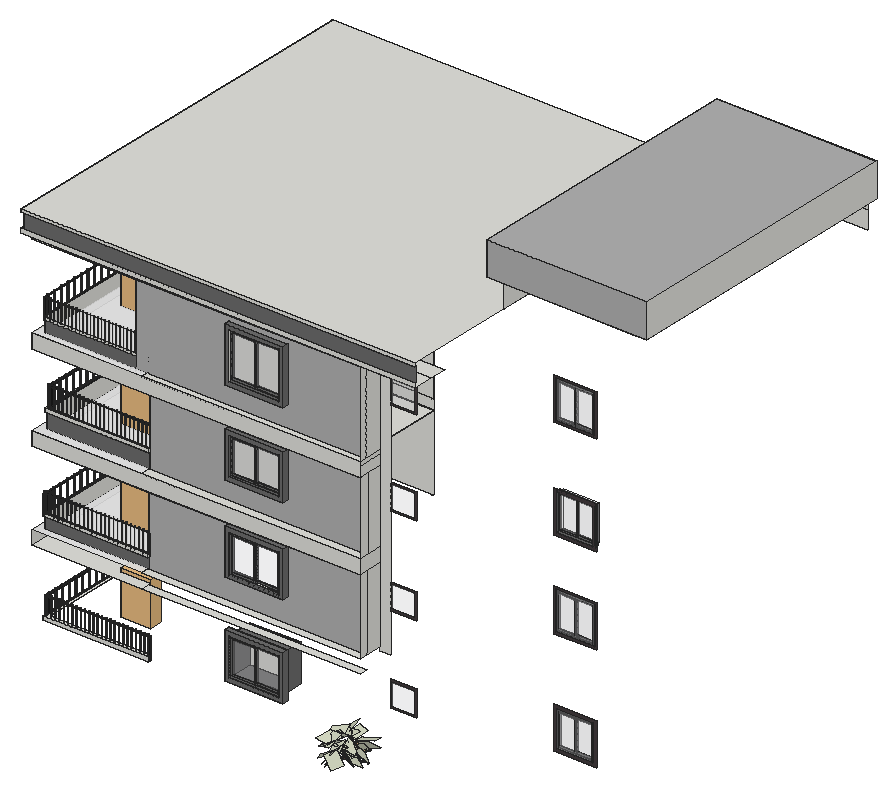
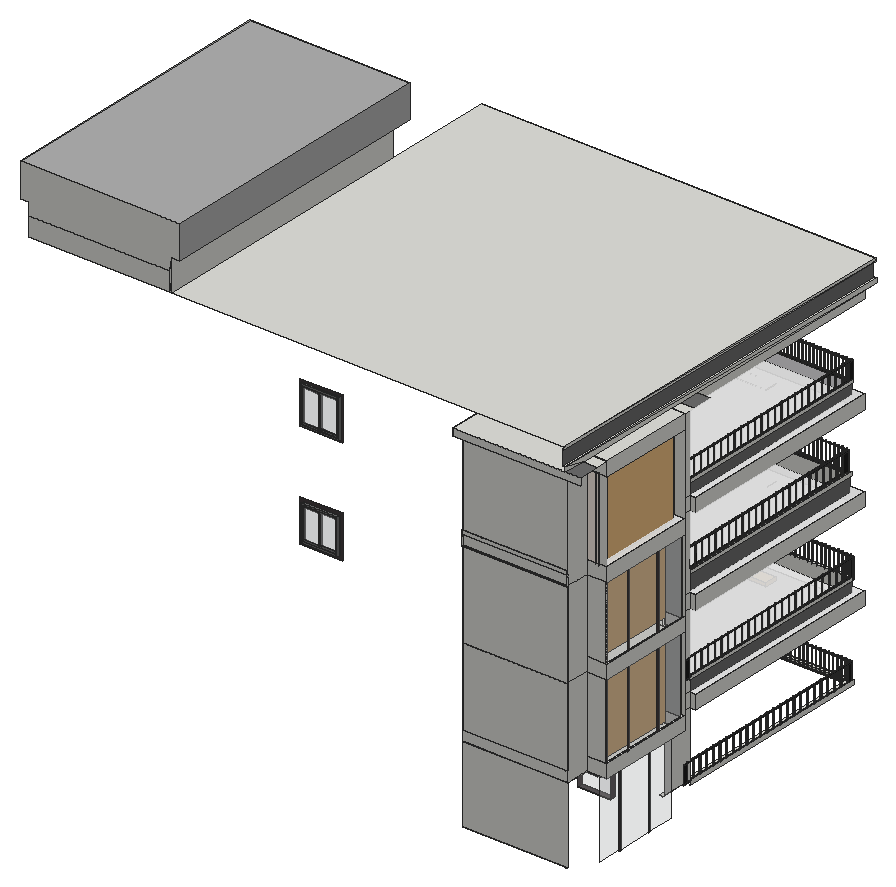
# SketchUp Ruby script. Lengths in inches.
U = 1.inch
M = Sketchup.active_model
def pt(a) = Geom::Point3d.new(a.map { |v| v * U })
def face(e, loops, mat)
  f = e.add_face(loops[0].map { |a| pt(a) })
  loops[1..].each { |l| e.add_face(l.map { |a| pt(a) }).erase! }
  f.material = f.back_material = mat if mat
  f
end
# faces: each face lists its corners as indices into pts; further lists are holes
def faces(e, pts, list, mat = nil) = list.each { |f| face(e, (f[0].is_a?(Array) ? f : [f]).map { |l| l.map { |i| pts[i] } }, mat) }
# xy, xz, yz: faces in a plane at the given z, y or x. An outline is a flat list of corners, or four numbers for a rectangle; further outlines are holes
def ring(l) = l.size == 4 ? [[l[0], l[1]], [l[2], l[1]], [l[2], l[3]], [l[0], l[3]]] : l.each_slice(2).to_a
def flat(e, list, mat, &to3) = list.each { |f| face(e, (f[0].is_a?(Array) ? f : [f]).map { |l| ring(l).map { |u, v| to3.(u, v) } }, mat) }
def xy(e, z, list, mat = nil) = flat(e, list, mat) { |x, y| [x, y, z] }
def xz(e, y, list, mat = nil) = flat(e, list, mat) { |x, z| [x, y, z] }
def yz(e, x, list, mat = nil) = flat(e, list, mat) { |y, z| [x, y, z] }
def lines(e, pts, list) = list.each { |a, b| e.add_line(pt(pts[a]), pt(pts[b])) }
# prism: a flat outline (further loops are holes) pulled along v
def prism(e, loops, v, mat = nil)
  f = face(e, loops, mat); d = Geom::Vector3d.new(v.map { |x| x * U })
  f.pushpull(f.normal.samedirection?(d) ? d.length : -d.length)
end
def box(e, o, s, mat = nil) = prism(e, [[o, [o[0] + s[0], o[1], o[2]], [o[0] + s[0], o[1] + s[1], o[2]], [o[0], o[1] + s[1], o[2]]]], [0, 0, s[2]], mat)
def at(x, y, z, deg = 0) = Geom::Transformation.translation(pt([x, y, z])) * Geom::Transformation.rotation(ORIGIN, Z_AXIS, deg.degrees)
def axes(o, x, y, z) = Geom::Transformation.new([*x, 0, *y, 0, *z, 0, *pt(o).to_a, 1])
def part(name) = M.definitions.add(name)
# library, detail: a bought-in or finely detailed component or shape, given as its bounding box
def library(name, o, s) = part(name).tap { |d| box(d.entities, o, s) }
def detail(e, o, s) = box(e.add_group.entities, o, s)
def put(e, d, t, mat = nil) = e.add_instance(d, t).tap { |i| i.material = mat if mat }
def group(e, t, mat = nil) = e.add_group.tap { |g| g.transformation = t; g.material = mat if mat }.entities
root = M.entities
M.materials.add("Celtis_australis_s cópia1").color = [224, 229, 205]
M.materials.add("Niraj_Hair_Dark").color = [109, 109, 109]
M.materials.add("Niraj_Hair_Gray").color = [178, 178, 178]
M.materials.add("Tendaggio").color = [239, 239, 239]
M.materials["Tendaggio"].alpha = 0.9
M.materials.add("[0009_Linen]").color = [250, 240, 230]
M.materials.add("[Asphalt New]").color = [67, 60, 62]
M.materials.add("[Color M08]").color = [30, 30, 30]
M.materials.add("[CoolGray4]").color = [225, 226, 230]
M.materials["[CoolGray4]"].alpha = 0.26
M.materials.add("aubin blanc").color = [238, 236, 240]
M.materials.add("bark_cherry").color = [99, 76, 62]
c1 = part("branch2\#1")
p = [[13.74,0.36,0.5],[11.5,11.3125,10.98],[14.125,0.95,0],[14.97,0.95,0.19],[12.12,10.6875,11.67],[15.1,0.36,0.82],
  [11.05,10.4375,11.49],[14.34,0,1.01],[6.08,18.54,23.51],[6.83,18.32,23.89],[6.09,17.93,24.13],[3.27,29.37,34],
  [3.27,29.68,33.56],[3.73,29.59,33.82],[0,43.16,40.74],[0,43.16,40.75],[0.01,43.16,40.75],[5.59,23.2,32.77],
  [4.65,30.48,39.08],[1.92,39.79,43.02],[5.09,28.47,41.41]]
faces(c1.entities,p,[[0,1,2],[2,1,3],[3,4,5],[3,1,4],[6,0,7],[0,6,1],[5,6,7],[6,5,4],
  [6,8,1],[1,9,4],[9,1,8],[8,6,10],[4,10,6],[10,4,9],[10,11,8],[8,12,9],
  [12,8,11],[10,9,11],[13,11,9],[13,9,12],[14,12,11,15],[12,14,16,13],[13,16,15,11]],"bark_cherry")
lines(c1.entities,p,[[17,18],[11,19],[20,17],[17,10]])
c2 = part("branch3")
p = [[6.085,7.082,2.644],[4.083,0.001,0],[4.08,0.002,0.001],[5.841,7.141,2.739],[4.083,0,0.004],[6.032,7.035,2.901],
  [8.234,14.378,3.666],[10.055,21.673,1.937],[8.611,14.241,3.496],[10.247,21.661,2.456],[9.737,21.9,2.346],[9.715,21.803,2.365],
  [12.357,28.999,2.225],[12.894,28.763,2.608],[12.761,28.844,2.204],[10.064,22.087,2.083],[10.362,21.9,2.346],[5.434,16.028,3.111],
  [10.04,22.14,2.516],[12.239,29.014,2.642],[8.553,14.232,3.928],[5.628,15.927,3.273],[5.444,16.098,3.367],[12.571,28.869,2.879],
  [0.628,10.534,6.01],[0.625,10.536,6.008],[0.625,10.537,6.012],[6.135,9.846,4.735],[0.003,10.534,6.01],[0,10.537,6.012],
  [1.761,10.232,4.093],[4.16,5.476,4.049],[3.718,5.459,5.543],[3.205,0.783,1.919]]
faces(c2.entities,p,[[0,1,2,3],[3,2,4,5],[1,0,5,4],[6,7,8],[9,8,7],[7,6,10,11],[12,7,11],[13,7,14],
  [14,7,12],[13,9,7],[15,16,17],[15,17,18],[12,11,19],[20,10,6],[10,20,9,11],[21,17,16],
  [21,16,22],[18,22,16],[9,19,11],[8,9,20],[22,18,17],[9,13,23],[19,9,23],[0,8,5],
  [3,6,0],[8,0,6],[3,5,6],[20,5,8],[20,6,5],[21,24,25,17],[26,22,17,25],[22,26,24,21]],"bark_cherry")
lines(c2.entities,p,[[27,20],[28,29],[17,30],[27,31],[32,27],[5,33]])
c3 = part("leaf1\#1")
p = [[1.6,6.78,0.04],[-9.34,-4.04,0.02],[2.67,-16.2,2.05],[13.62,-5.38,2.07]]
faces(c3.entities,p,[[0,1,2,3]],"Celtis_australis_s cópia1")
c4 = part("leaf_group1\#1")
put(c4.entities,c3,axes([-0.06,3.68,7.3125],[0.53029,-0.80282,-0.27253],[0.82812,0.42159,0.36943],[-0.18168,-0.42159,0.8884]))
put(c4.entities,c3,axes([6.4375,-3.58,5.23],[1,0,0],[0,0.98927,0.14608],[0,-0.14608,0.98927]))
put(c4.entities,c3,axes([-0.99,3.68,1.22],[0.57591,-0.80282,0.15431],[0.36532,0.42159,0.82994],[-0.73135,-0.42159,0.53609]))
put(c4.entities,c3,axes([18.71,8.59,4.39],[0.33053,0.77491,0.53877],[-0.79988,-0.073,0.5957],[0.50094,-0.62785,0.5957]))
put(c4.entities,c3,axes([13.16,0.76,0.89],[0.89618,0.3501,0.27256],[-0.44248,0.65988,0.60727],[0.03275,-0.66482,0.74628]))
put(c4.entities,c3,axes([4.53,7.98,7.3125],[-0.1927,0.94265,-0.27253],[0.88368,0.28746,0.36943],[-0.42658,0.16964,0.8884]))
put(c4.entities,c3,axes([12.46,21.28,7.16],[0.85019,0.38493,0.35918],[0.30538,-0.91629,0.25914],[-0.42887,0.11063,0.89657]))
put(c4.entities,c3,axes([6.53,15.18,2.59],[0.70711,0.70711,0],[0.5,-0.5,0.70711],[-0.5,0.5,0.70711]))
put(c4.entities,c3,axes([-3.17,8.15,3.46],[-0.03719,0.74973,0.66069],[0.94096,-0.19634,0.27576],[-0.33647,-0.63194,0.69817]))
put(c4.entities,c3,axes([23.03,17.79,4.39],[0.78166,-0.31422,0.53877],[-0.61722,-0.51398,0.5957],[-0.08973,0.79818,0.5957]))
put(c4.entities,c3,axes([14.78,21.52,3.21],[0.67246,-0.04394,0.73882],[-0.28657,-0.93583,0.20517],[-0.6824,0.3497,0.64191]))
put(c4.entities,c3,axes([10.37,-1.8125,9],[0.99279,-0.06448,-0.101],[0.11527,0.74421,0.65792],[0.03275,-0.66482,0.74628]))
put(c4.entities,c3,axes([1.45,16.1875,2.9375],[-0.2106,-0.86579,-0.45394],[0.96054,-0.26957,0.06852],[-0.18168,-0.42159,0.8884]))
c5 = part("branch1\#1")
p = [[23.875,19.65,51.47],[23.47,20.4,51.62],[21.1,21.64,19.5],[21.93,21.1875,19.92],[21.95,22.18,19.69],[26.48,9.62,42.86],
  [30.79,16.22,49.68],[31.01,4.77,55.38],[31.01,0,68.57],[9.91,24.21,59.69],[9.92,24.21,59.7],[24,20.54,51.64],
  [12.85,4.92,53.79],[26.1,8.92,42.74],[31.84,25.13,88.91],[31.84,25.13,106.45],[30.18,33.29,93.95],[30.18,25.42,69.53],
  [0,6.37,81.52],[11.1,10.75,77.87]]
lines(c5.entities,p,[[0,1],[2,3],[3,4],[5,6],[7,8],[9,10],[1,11],[11,0],[12,13],[4,2],[14,15],[16,17],
  [18,19]])
detail(c5.entities,[5.26,2.24,0],[28.14,24.14,108.01])
c6 = part("Group\#428")
prism(c6.entities,[[[0,1.97,0],[0,1.97,1.18],[0,0,1.18],[0,0,0]],[[0,1.92,1.13],[0,1.92,0.05],[0,0.05,0.05],[0,0.05,1.13]]],[98.43,0,0])
c7 = part("Group\#430")
xy(c7.entities,0,[[0.3,0,0.22,0.01,0.15,0.04,0.09,0.09,0.04,0.15,0.01,0.22,0,0.3,0.3,0.3],[0.3,0,0.3,0.3,0.59,0.3,0.58,0.22,0.55,0.15,0.5,0.09,0.44,0.04,0.37,0.01],[0,0.3,0.01,0.37,0.04,0.44,0.09,0.5,0.15,0.55,0.22,0.58,0.3,0.59,0.3,0.3],[0.3,0.3,0.3,0.59,0.37,0.58,0.44,0.55,0.5,0.5,0.55,0.44,0.58,0.37,0.59,0.3]])
xy(c7.entities,39.37,[[0.3,0,0.37,0.01,0.44,0.04,0.5,0.09,0.55,0.15,0.58,0.22,0.59,0.3,0.58,0.37,0.55,0.44,0.5,0.5,0.44,0.55,0.37,0.58,0.3,0.59,0.22,0.58,0.15,0.55,0.09,0.5,0.04,0.44,0.01,0.37,0,0.3,0.01,0.22,0.04,0.15,0.09,0.09,0.15,0.04,0.22,0.01]])
p = [[0.09,0.09,0],[0.15,0.04,0],[0.15,0.04,39.37],[0.09,0.09,39.37],[0.22,0.01,0],[0.22,0.01,39.37],
  [0.3,0,0],[0.3,0,39.37],[0.37,0.01,0],[0.37,0.01,39.37],[0.44,0.04,0],[0.44,0.04,39.37],
  [0.5,0.09,0],[0.5,0.09,39.37],[0.01,0.22,0],[0.04,0.15,0],[0.04,0.15,39.37],[0.01,0.22,39.37],
  [0.55,0.15,0],[0.55,0.15,39.37],[0.58,0.22,0],[0.58,0.22,39.37],[0,0.3,0],[0,0.3,39.37],
  [0.59,0.3,0],[0.59,0.3,39.37],[0.01,0.37,0],[0.01,0.37,39.37],[0.58,0.37,0],[0.58,0.37,39.37],
  [0.09,0.5,0],[0.04,0.44,0],[0.04,0.44,39.37],[0.09,0.5,39.37],[0.55,0.44,0],[0.5,0.5,0],
  [0.5,0.5,39.37],[0.55,0.44,39.37],[0.15,0.55,0],[0.15,0.55,39.37],[0.44,0.55,0],[0.44,0.55,39.37],
  [0.22,0.58,0],[0.22,0.58,39.37],[0.3,0.59,0],[0.3,0.59,39.37],[0.37,0.58,0],[0.37,0.58,39.37]]
faces(c7.entities,p,[[0,1,2,3],[1,4,5,2],[4,6,7,5],[6,8,9,7],[8,10,11,9],[10,12,13,11],[14,15,16,17],[15,0,3,16],
  [12,18,19,13],[18,20,21,19],[22,14,17,23],[20,24,25,21],[26,22,23,27],[24,28,29,25],[30,31,32,33],[31,26,27,32],
  [34,35,36,37],[28,34,37,29],[38,30,33,39],[35,40,41,36],[42,38,39,43],[44,42,43,45],[46,44,45,47],[40,46,47,41]])
c8 = part("Group\#429")
prism(c8.entities,[[[0.01,0.22,35.83],[0,0.3,35.83],[0.01,0.37,35.83],[0.04,0.44,35.83],[0.09,0.5,35.83],[0.15,0.55,35.83],[0.22,0.58,35.83],[0.3,0.59,35.83],[0.37,0.58,35.83],[0.44,0.55,35.83],[0.5,0.5,35.83],[0.55,0.44,35.83],[0.58,0.37,35.83],[0.59,0.3,35.83],[0.58,0.22,35.83],[0.55,0.15,35.83],[0.5,0.09,35.83],[0.44,0.04,35.83],[0.37,0.01,35.83],[0.3,0,35.83],[0.22,0.01,35.83],[0.15,0.04,35.83],[0.09,0.09,35.83],[0.04,0.15,35.83]]],[0,0,3.54])
c9 = part("Balcony railing panel")
g1 = group(c9.entities,at(0,0,0))
put(g1,c6,axes([0,0,39.76],[1,0,0],[0,0,-1],[0,1,0]),"[Color M08]")
put(g1,c6,axes([0,0,1.97],[1,0,0],[0,0,-1],[0,1,0]),"[Color M08]")
put(g1,c6,axes([98.43,0,37.8],[0,0,-0.364],[-1,0,0],[0,1,0]),"[Color M08]")
put(g1,c6,axes([1.97,0,37.8],[0,0,-0.364],[-1,0,0],[0,1,0]),"[Color M08]")
g2 = group(c9.entities,at(1.67,0.3,1.97))
put(g2,c7,at(78.74,0,0),"[Color M08]")
put(g2,c7,at(90.55,0,0),"[Color M08]")
put(g2,c7,at(82.68,0,0),"[Color M08]")
put(g2,c7,at(86.61,0,0),"[Color M08]")
put(g2,c7,at(66.93,0,0),"[Color M08]")
put(g2,c7,at(11.8125,0,0),"[Color M08]")
put(g2,c7,at(15.75,0,0),"[Color M08]")
put(g2,c7,at(47.24,0,0),"[Color M08]")
put(g2,c7,at(59.06,0,0),"[Color M08]")
put(g2,c8,at(0,0,0),"[Color M08]")
put(g2,c7,at(39.37,0,0),"[Color M08]")
put(g2,c7,at(62.99,0,0),"[Color M08]")
put(g2,c7,at(55.12,0,0),"[Color M08]")
put(g2,c7,at(19.69,0,0),"[Color M08]")
put(g2,c7,at(35.43,0,0),"[Color M08]")
put(g2,c7,at(7.875,0,0),"[Color M08]")
put(g2,c7,at(23.62,0,0),"[Color M08]")
put(g2,c7,at(31.5,0,0),"[Color M08]")
put(g2,c7,at(43.31,0,0),"[Color M08]")
put(g2,c7,at(27.56,0,0),"[Color M08]")
put(g2,c7,at(3.9375,0,0),"[Color M08]")
put(g2,c7,at(51.18,0,0),"[Color M08]")
put(g2,c7,at(70.87,0,0),"[Color M08]")
put(g2,c7,at(74.8,0,0),"[Color M08]")
put(g2,c8,at(94.49,0,0),"[Color M08]")
c10 = part("Window sash")
g3 = group(c10.entities,at(0.98,0,0),"Niraj_Hair_Dark")
prism(g3,[[[-0.98,0,0],[30.98,0,0],[30.98,0,45.6],[-0.98,0,45.6]],[[29.01,0,43.625],[29.01,0,1.97],[0.98,0,1.97],[0.98,0,43.625]]],[0,1.18,0])
g4 = group(c10.entities,at(1.97,0.59,1.97))
xz(g4,0,[[0,0,28.03,41.66]],"[CoolGray4]")
c11 = part("Twin sash window")
put(c11.entities,c10,at(31.97,2.82,1.97))
put(c11.entities,c10,at(1.97,1.25,1.97))
g5 = group(c11.entities,at(0,0,0),"Niraj_Hair_Dark")
prism(g5,[[[65.9,4.72,0],[0,4.72,0],[0,4.72,49.53],[65.9,4.72,49.53]],[[1.97,4.72,47.5625],[1.97,4.72,1.97],[63.93,4.72,1.97],[63.93,4.72,47.5625]]],[0,-4.72,0])
c12 = library("Plane01\#1",[-62.23,-4.43,-95.54],[61.02,8.86,95.65])
c13 = library("Tenda",[0,0,0],[9.09,66.93,111.26])
c14 = library("fronceur+aubin+blanc+(3)",[-47.99,-0.29,1.66],[95.37,4.84,114.09])
xy(root,221.21,[[544.51,339.47,577.96,344.47]],"[Asphalt New]")
xy(root,224.0625,[[500.29,454.11,605.23,454.18]])
xy(root,231.41,[[499.48,97,499.48,301.21,500.29,301.21,500.29,97.6875,605.23,97.6875,605.23,97]])
xy(root,235.75,[[499.48,97,605.23,97,605.23,100.3125,503.33,100.3125,503.33,335.4,500.29,335.4,500.29,301.21,499.48,301.21]])
xy(root,245.54,[[686.26,91.1875,745.01,96.375]],"Niraj_Hair_Dark")
xy(root,249.54,[[690.26,91.1875,741.01,118.125]],"Niraj_Hair_Dark")
xy(root,285,[[544.51,339.47,577.96,344.47]],"[Asphalt New]")
xy(root,287.23,[[690.26,91.1875,741.01,118.125]],"Niraj_Hair_Dark")
xy(root,287.65,[[541.86,336.16,580.61,339.47]])
xy(root,291.23,[[686.26,91.1875,745.01,96.375]],"Niraj_Hair_Dark")
xy(root,299.625,[[488.54,336.16,605.23,336.16,605.23,454.11,500.29,454.11,500.29,430.89,488.54,430.89]])
xy(root,300.47,[[494.79,89.375,494.79,301.21,500.29,301.21,500.29,333.01,479.54,333.01,479.54,430.89,500.29,430.89,500.29,454.11,605.23,454.11,605.23,89.375],[605.23,89.375,823.9,97.6875]])
xy(root,310.625,[[500.29,454.11,605.23,454.49]])
xy(root,314.1875,[[605.23,89.375,823.9,97.3125]])
xy(root,314.1875,[[494.79,89.375,605.23,89.375,605.23,97.3125,500.73,97.3125,500.73,301.21,502.61,301.21,502.61,98.8125,605.23,98.8125,605.23,336.16,580.61,336.16,580.61,341.72,541.86,341.72,541.86,336.16,481.17,336.16,481.17,430.89,479.54,430.89,479.54,333.01,500.29,333.01,500.29,301.21,494.79,301.21]],"Tendaggio")
xy(root,325.23,[[499.98,96.5,605.23,97.3125],[499.98,97.3125,500.73,301.21]])
xy(root,328.3125,[[499.98,96.5,605.23,96.5,605.23,98.8125,502.61,98.8125,502.61,301.21,499.98,301.21]])
xy(root,338.8,[[686.26,91.1875,745.01,96.375]],"Niraj_Hair_Dark")
xy(root,342.8,[[690.26,91.1875,741.01,97.3125]])
xy(root,380.29,[[690.26,91.1875,741.01,97.3125]])
xy(root,381.08,[[541.86,336.16,580.61,341.72]])
xy(root,384.29,[[686.26,91.1875,745.01,96.375]],"Niraj_Hair_Dark")
xy(root,389.4,[[494.79,89.375,494.79,301.21,500.29,301.21,500.29,333.01,479.54,333.01,479.54,430.89,481.17,430.89,481.17,336.16,605.23,336.16,605.23,89.375],[605.23,89.375,823.9,97.3125],[605.23,97.3125,823.9,113.9375],[481.17,336.16,605.23,336.16,605.23,454.11,500.29,454.11,500.29,430.89,481.17,430.89],[500.29,454.11,605.23,454.49]])
xy(root,403.5,[[605.23,89.375,823.9,98.6875],[605.23,98.6875,823.9,113.9375]])
xy(root,403.5,[[494.79,89.375,605.23,89.375,605.23,98.6875,501.67,98.6875,501.67,301.21,502.78,301.21,502.78,99.8125,605.23,99.8125,605.23,336.16,580.61,336.16,580.61,338.78,541.86,338.78,541.86,336.16,480.73,336.16,480.73,430.89,479.54,430.89,479.54,333.01,500.29,333.01,500.29,301.21,494.79,301.21]],"Tendaggio")
xy(root,404.95,[[543.31,338.78,579.16,338.78,579.16,339.47],[543.31,338.78,579.16,339.47,543.31,339.47]],"[Asphalt New]")
xy(root,419.01,[[501.11,97.6875,501.67,301.21],[501.67,97.6875,605.23,98.6875]])
xy(root,422.125,[[501.11,97.6875,605.23,97.6875,605.23,99.8125,502.78,99.8125,502.78,301.21,501.11,301.21]])
xy(root,425.67,[[686.26,91.1875,745.01,96.375]],"Niraj_Hair_Dark")
xy(root,426.12,[[942.54,187.625,978.5,195.5]],"[CoolGray4]")
xy(root,429.67,[[690.26,91.1875,741.01,96.375]])
xy(root,462.08,[[942.54,187.625,978.5,195.5]],"[CoolGray4]")
xy(root,466.04,[[543.31,338.78,543.31,339.47,579.16,339.47],[543.31,338.78,579.16,339.47,579.16,338.78]],"[Asphalt New]")
xy(root,467.36,[[690.26,91.1875,741.01,96.375]],"Niraj_Hair_Dark")
xy(root,467.49,[[541.86,336.16,580.61,338.78]],"[Asphalt New]")
xy(root,471.36,[[686.26,91.1875,745.01,96.375]],"Niraj_Hair_Dark")
xy(root,476.89,[[494.79,89.375,494.79,301.21,500.29,301.21,500.29,333.01,479.54,333.01,479.54,430.89,480.73,430.89,480.73,336.16,605.23,336.16,605.23,89.375],[605.23,89.375,823.9,98.6875],[605.23,98.6875,823.9,113.9375],[480.73,336.16,605.23,336.16,605.23,454.49,500.29,454.49,500.29,430.89,480.73,430.89],[500.29,454.49,605.23,455.3]])
xy(root,490.8125,[[605.23,89.375,823.9,96.375],[605.23,96.375,823.9,96.375,823.9,113.9375,593.42,113.9375,593.42,96.75,605.23,96.75],[593.42,113.9375,605.23,336.16],[500.29,454.49,605.23,455.3]])
xy(root,490.8125,[[494.79,89.375,605.23,89.375,605.23,96.375,501.48,96.375,501.48,303.8125,502.03,303.8125,502.03,96.75,593.42,96.75,593.42,336.16,580.61,336.16,580.61,342.78,541.86,342.78,541.86,336.16,488.04,336.16,488.04,430.89,479.54,430.89,479.54,333.01,500.29,333.01,500.29,301.21,494.79,301.21]],"Tendaggio")
xy(root,501.26,[[500.54,302.0625,501.48,303.3125],[500.54,303.3125,501.48,303.8125]])
xy(root,501.76,[[500.54,96.375,501.48,302.0625]])
xy(root,504.625,[[500.54,96.375,593.42,96.375,593.42,96.75,502.03,96.75,502.03,303.8125,500.54,303.8125]])
xy(root,510.98,[[686.26,91.1875,745.01,96.375]],"Niraj_Hair_Dark")
xy(root,514.98,[[690.26,91.1875,741.01,96.375]])
xy(root,562.11,[[690.26,91.1875,741.01,96.375]])
xy(root,566.11,[[686.26,91.1875,745.01,96.375]],"Niraj_Hair_Dark")
xy(root,566.625,[[541.86,336.16,580.61,342.78]])
xy(root,571.4375,[[479.54,333.01,500.29,333.01,500.29,336.16,488.04,336.16,488.04,430.89,479.54,430.89]])
xy(root,571.4375,[[488.04,336.16,500.29,430.89]],"[0009_Linen]")
xy(root,575.91,[[494.79,89.375,494.79,301.21,500.29,301.21,500.29,336.16,593.42,336.16,593.42,96.375,605.23,96.375,605.23,89.375],[605.23,89.375,823.9,96.375],[593.42,96.375,823.9,113.9375],[593.42,113.9375,605.23,336.16]])
xy(root,585.8125,[[493.11,76.75,493.11,96.75,494.79,96.75,494.79,89.375,582.17,89.375,582.17,76.75],[582.17,76.75,605.23,89.375],[605.23,76.75,605.23,89.375,834.53,89.375,834.53,96.75,888.71,96.75,888.71,76.75],[494.79,89.375,605.23,89.375,605.23,113.9375,607.36,464.11,495.23,464.11,493.11,443.75,493.11,430.89,500.29,430.89,500.29,333.01,493.11,333.01,493.11,301.21,494.79,301.21],[605.23,89.375,834.53,113.9375],
  [493.11,96.75,494.79,301.21],[834.53,96.75,888.71,113.9375],[479.54,321.37,493.11,333.01],[479.54,333.01,493.11,430.89],[493.11,333.01,500.29,430.89],
  [479.54,430.89,493.11,443.75]])
xy(root,585.8125,[[479.54,301.21,493.11,321.37],[479.54,443.75,493.11,443.75,495.23,464.11,479.54,464.11]],"Niraj_Hair_Dark")
xy(root,590.04,[[493.11,76.75,580.54,76.75,580.54,77.375,495.67,77.375,497.79,464.11,495.23,464.11],[580.54,76.75,888.71,77.375]])
xy(root,604.78,[[493.79,76.75,580.54,77.375],[580.54,76.75,888.71,77.375],[493.79,77.375,495.92,464.11,497.79,464.11,495.67,77.375]])
xy(root,607.875,[[493.79,76.75,888.71,76.75,888.71,464.11,495.92,464.11],[888.71,187.625,890.84,464.11,888.71,464.11]])
xy(root,639.04,[[881.03,176.0625,888.71,464.11],[888.71,176.0625,888.71,187.625,1032.97,187.625,1030.84,176.0625],[1030.84,176.0625,1032.97,187.625,1032.97,464.11,1041.03,464.11,1041.03,176.0625]])
xy(root,672.6875,[[881.03,176.0625,1041.03,464.11]],"Niraj_Hair_Gray")
xz(root,76.75,[[493.11,585.8125,888.71,590.04],[493.79,604.78,888.71,607.875]])
xz(root,77.375,[[495.67,590.04,888.71,604.78]],"Niraj_Hair_Dark")
xz(root,89.375,[[494.79,389.4,823.9,403.5],[494.79,476.89,823.9,490.8125]])
xz(root,91.1875,[[[686.26,245.54,745.01,291.23],[690.26,249.54,741.01,287.23]],[[686.26,338.8,745.01,384.29],[690.26,342.8,741.01,380.29]],[[686.26,425.67,745.01,471.36],[690.26,429.67,741.01,467.36]],[[686.26,510.98,745.01,566.11],[690.26,514.98,741.01,562.11]]],"Niraj_Hair_Dark")
xz(root,96.375,[[[686.26,245.54,745.01,291.23],[690.26,249.54,741.01,287.23]],[[686.26,338.8,745.01,384.29],[690.26,342.8,741.01,380.29]],[[686.26,425.67,745.01,471.36],[690.26,429.67,741.01,467.36]],[690.26,429.67,741.01,467.36],[500.54,501.76,593.42,504.625],
  [690.26,514.98,741.01,562.11]])
xz(root,96.375,[[501.48,490.8125,593.42,501.76]],"Niraj_Hair_Dark")
xz(root,96.375,[[[593.42,490.8125,823.9,575.91],[686.26,510.98,745.01,566.11]]],"Niraj_Hair_Gray")
xz(root,96.5,[[499.98,325.23,605.23,328.3125]])
xz(root,96.75,[[593.42,490.8125,605.23,504.625]])
xz(root,96.75,[[502.03,490.8125,593.42,504.625]],"aubin blanc")
xz(root,97,[[499.48,231.41,605.23,235.75]])
xz(root,97.3125,[[500.73,314.1875,605.23,325.23]],"Niraj_Hair_Dark")
xz(root,97.3125,[[[605.23,314.1875,823.9,389.4],[690.26,342.8,741.01,380.29]]],"Niraj_Hair_Gray")
xz(root,97.6875,[[501.11,419.01,605.23,422.125]])
xz(root,98.6875,[[501.67,403.5,605.23,419.01]],"Niraj_Hair_Dark")
xz(root,98.6875,[[605.23,403.5,823.9,476.89]],"Niraj_Hair_Gray")
xz(root,98.8125,[[502.61,314.1875,605.23,328.3125]])
xz(root,99.8125,[[502.78,403.5,605.23,422.125]])
xz(root,113.9375,[[823.9,310.625,823.9,575.91,605.23,575.91,605.23,585.8125,834.53,585.8125,834.53,310.625],[605.23,389.4,823.9,403.5],[605.23,476.89,823.9,487.5],[605.23,487.5,823.9,490.8125]])
xz(root,113.9375,[[[834.53,263.07,860.28,288.82],[836.11,264.65,858.7,287.24]],[[834.53,350.5,860.28,376.25],[836.11,352.09,858.7,374.67]],[[834.53,440.38,860.28,466.13],[835.75,441.6,859.05,464.91]],[[834.53,535.34,860.28,561.09],[835.875,536.69,858.93,559.75]]],"[Asphalt New]")
xz(root,113.9375,[[836.11,264.65,858.7,287.24],[836.11,352.09,858.7,374.67],[835.75,441.6,859.05,464.91],[835.875,536.69,858.93,559.75]],"[CoolGray4]")
xz(root,118.125,[[690.26,249.54,741.01,287.23]])
xz(root,176.0625,[[881.03,639.04,1041.03,672.6875]],"Niraj_Hair_Gray")
xz(root,187.625,[[[939.31,228.57,981.74,271],[942.54,231.8,978.5,267.76]],[[939.31,334.38,981.74,376.82],[941.35,336.42,979.7,374.77]],[[939.31,422.88,981.74,465.32],[942.54,426.12,978.5,462.08]],[[939.31,523.94,981.74,566.38],[941.18,525.81,979.875,564.51]]],"[Asphalt New]")
xz(root,187.625,[[942.54,231.8,978.5,267.76],[941.35,336.42,979.7,374.77],[941.18,525.81,979.875,564.51]],"[CoolGray4]")
xz(root,195.5,[[942.54,426.12,978.5,462.08]],"[CoolGray4]")
xz(root,301.21,[[494.79,300.47,500.29,314.1875],[500.73,314.1875,500.73,325.23,500.29,325.23,500.29,328.3125,502.61,328.3125,502.61,314.1875],[499.98,325.23,500.29,328.3125],[494.79,389.4,500.29,403.5],[501.67,403.5,501.67,419.01,501.11,419.01,501.11,422.125,502.78,422.125,502.78,403.5],
  [494.79,476.89,500.29,490.8125]])
xz(root,302.0625,[[500.54,501.26,501.48,501.76]])
xz(root,303.8125,[[501.48,490.8125,501.48,501.26,500.54,501.26,500.54,504.625,502.03,504.625,502.03,490.8125]])
xz(root,333.01,[[479.54,300.47,500.29,314.1875],[479.54,314.1875,500.29,389.4],[479.54,389.4,500.29,403.5],[479.54,403.5,500.29,476.89],[479.54,476.89,500.29,490.8125],
  [479.54,490.8125,500.29,571.4375],[479.54,571.4375,500.29,585.8125]])
xz(root,336.16,[[593.42,490.8125,605.23,575.91]])
xz(root,336.16,[[481.17,314.1875,541.86,314.1875,541.86,381.08,580.61,381.08,580.61,314.1875,605.23,314.1875,605.23,389.4,481.17,389.4],[480.73,403.5,541.86,403.5,541.86,467.49,580.61,467.49,580.61,403.5,605.23,403.5,605.23,476.89,480.73,476.89],[488.04,490.8125,541.86,490.8125,541.86,566.625,580.61,566.625,580.61,490.8125,593.42,490.8125,593.42,575.91,500.29,575.91,500.29,571.4375,488.04,571.4375]],"Niraj_Hair_Gray")
xz(root,338.78,[[541.86,403.5,563.23,403.5,558.66,404.95,543.31,404.95,543.31,466.04,579.16,466.04,579.16,404.95,558.66,404.95,563.23,403.5,580.61,403.5,580.61,467.49,541.86,467.49]],"[Asphalt New]")
xz(root,341.72,[[[541.86,314.1875,580.61,381.08],[543.32,315.65,579.15,379.62]]],"[Asphalt New]")
xz(root,342.78,[[[541.86,490.8125,580.61,566.625],[543.75,492.7,578.72,564.73]]],"[Asphalt New]")
xz(root,342.78,[[543.75,492.7,566.83,564.73],[566.83,492.7,578.72,564.73]],"[CoolGray4]")
xz(root,344.47,[[544.51,221.21,577.96,285]],"[CoolGray4]")
xz(root,430.89,[[479.54,300.47,500.29,314.1875],[479.54,314.1875,481.17,389.4],[481.17,314.1875,500.29,389.4],[479.54,389.4,500.29,403.5],[479.54,403.5,480.73,476.89],
  [480.73,403.5,500.29,476.89],[479.54,476.89,500.29,490.8125],[479.54,490.8125,488.04,571.4375],[479.54,571.4375,500.29,585.8125]])
xz(root,430.89,[[488.04,490.8125,500.29,571.4375]],"[0009_Linen]")
xz(root,454.11,[[500.29,224.0625,605.23,299.625],[500.29,299.625,605.23,300.47],[500.29,300.47,605.23,310.625],[500.29,310.625,605.23,389.4]])
xz(root,454.49,[[500.29,310.625,605.23,389.4],[500.29,389.4,605.23,476.89],[500.29,476.89,605.23,490.8125],[500.29,490.8125,605.23,575.91]])
xz(root,455.3,[[500.29,487.5,605.23,490.8125]])
xz(root,464.11,[[479.54,578.41,607.36,585.8125],[888.71,607.875,888.71,639.04,890.84,607.875],[890.84,607.875,890.84,626.48,888.71,639.04],[890.84,607.875,1032.97,626.48],[890.84,626.48,888.71,639.04,881.03,639.04,881.03,672.6875,1041.03,672.6875,1041.03,639.04,1032.97,639.04,1032.97,626.48]])
yz(root,479.54,[[333.01,300.47,430.89,314.1875],[333.01,389.4,430.89,403.5],[333.01,476.89,430.89,490.8125],[333.01,571.4375,430.89,585.8125]])
yz(root,479.54,[[366.65,314.1875,368.36,389.4],[404.03,314.1875,405.53,389.4],[366.65,403.5,368.36,476.89],[404.03,403.5,405.53,476.89]],"[Asphalt New]")
yz(root,480.73,[[336.16,403.5,430.89,476.89]],"[CoolGray4]")
yz(root,481.17,[[336.16,314.1875,430.89,389.4]],"[CoolGray4]")
yz(root,488.04,[[336.16,490.8125,336.16,571.4375,383.52,571.4375,383.52,570.03,337.57,570.03,337.57,492.22,383.52,492.22,383.52,490.8125],[383.52,490.8125,383.52,492.22,429.48,492.22,429.48,570.03,383.52,570.03,383.52,571.4375,430.89,571.4375,430.89,490.8125],[367.95,492.22,368.75,570.03],[404.54,492.22,405.66,570.03]],"[Asphalt New]")
yz(root,488.04,[[337.57,492.22,367.95,570.03],[368.75,492.22,404.54,570.03],[405.66,492.22,429.48,570.03]],"[CoolGray4]")
yz(root,488.54,[[365.75,220.95,367.47,297.24],[402.66,220.95,403.13,297.24],[403.13,220.95,404.63,297.24]],"[Asphalt New]")
yz(root,488.54,[[338.54,220.95,365.75,297.24],[367.47,220.95,402.66,297.24],[404.63,220.95,428.5,297.24]],"[CoolGray4]")
yz(root,493.79,[[76.75,604.78,76.75,607.875,77.375,604.78]])
yz(root,494.79,[[89.375,300.47,301.21,314.1875],[89.375,389.4,301.21,403.5],[89.375,476.89,301.21,490.8125],[89.375,575.91,301.21,585.8125]])
yz(root,499.48,[[97,231.41,301.21,235.75]])
yz(root,499.98,[[96.5,325.23,301.21,328.3125]])
yz(root,500.29,[[301.21,235.75,333.01,300.47],[430.89,299.625,454.11,300.47],[301.21,300.47,333.01,314.1875],[430.89,300.47,454.11,389.4],[454.11,310.625,454.49,389.4],
  [301.21,314.1875,333.01,389.4],[301.21,389.4,333.01,403.5],[430.89,389.4,454.43,476.89],[454.43,389.4,454.49,476.89],[301.21,403.5,333.01,476.89],
  [301.21,476.89,333.01,490.8125],[430.89,476.89,454.49,575.91],[454.49,476.89,455.3,487.5],[454.49,487.5,455.3,490.8125],[301.21,490.8125,333.01,575.91],
  [333.01,571.4375,336.16,575.91],[336.16,571.4375,430.89,575.91],[333.01,575.91,430.89,585.8125]])
yz(root,500.54,[[302.0625,501.26,302.0625,501.76,96.375,501.76,96.375,504.625,303.8125,504.625,303.8125,501.26]])
yz(root,500.73,[[97.3125,314.1875,301.21,325.23]],"Niraj_Hair_Dark")
yz(root,501.11,[[97.6875,419.01,301.21,422.125]])
yz(root,501.48,[[96.375,490.8125,96.375,501.76,302.0625,501.76,302.0625,501.26,303.8125,501.26,303.8125,490.8125]],"Niraj_Hair_Dark")
yz(root,501.67,[[98.6875,403.5,301.21,419.01]],"Niraj_Hair_Dark")
yz(root,502.03,[[96.75,490.8125,303.8125,504.625]])
yz(root,502.61,[[98.8125,314.1875,301.21,328.3125]])
yz(root,502.78,[[99.8125,403.5,301.21,422.125]])
yz(root,541.86,[[336.16,314.1875,341.72,381.08],[336.16,490.8125,342.78,566.625]])
yz(root,541.86,[[336.16,403.5,338.78,467.49]],"[Asphalt New]")
yz(root,543.31,[[338.78,404.95,339.47,466.04]],"[Asphalt New]")
yz(root,544.51,[[339.47,221.21,344.47,285]],"[Asphalt New]")
yz(root,577.96,[[339.47,221.21,344.47,285]],"[Asphalt New]")
yz(root,579.16,[[338.78,404.95,339.47,466.04]],"[Asphalt New]")
yz(root,580.61,[[336.16,314.1875,341.72,381.08],[336.16,403.5,338.78,467.49],[336.16,490.8125,342.78,566.625]],"[Asphalt New]")
yz(root,593.42,[[96.75,490.8125,96.75,504.625,96.375,504.625,96.375,575.91,336.16,575.91,336.16,490.8125]])
yz(root,605.23,[[97,231.41,97.6875,235.75],[454.11,310.625,454.49,389.4],[98.8125,314.1875,98.8125,328.3125,97.3125,328.3125,97.3125,389.4,336.16,389.4,336.16,314.1875],[96.5,325.23,97.3125,328.3125],[113.9375,389.4,113.9375,403.5,336.16,403.5,336.16,476.89,454.49,476.89,454.49,389.4],
  [98.6875,403.5,99.8125,422.125],[99.8125,403.5,99.8125,422.125,98.6875,422.125,98.6875,476.89,336.16,476.89,336.16,403.5],[97.6875,419.01,98.6875,422.125],[113.9375,476.89,454.49,487.5],[454.49,476.89,455.3,487.5],
  [113.9375,487.5,113.9375,490.8125,336.16,490.8125,336.16,575.91,454.49,575.91,454.49,487.5],[454.49,487.5,455.3,490.8125],[113.9375,575.91,113.9375,585.8125,336.16,575.91],[336.16,575.91,454.49,578.41,454.49,575.91]])
yz(root,686.26,[[91.1875,425.67,96.375,471.36]])
yz(root,686.26,[[91.1875,245.54,96.375,291.23],[91.1875,338.8,96.375,384.29],[91.1875,510.98,96.375,566.11]],"Niraj_Hair_Dark")
yz(root,690.26,[[91.1875,342.8,97.3125,380.29],[91.1875,514.98,96.375,562.11]])
yz(root,690.26,[[91.1875,249.54,118.125,287.23],[91.1875,429.67,96.375,467.36]],"Niraj_Hair_Dark")
yz(root,741.01,[[91.1875,342.8,97.3125,380.29],[91.1875,429.67,96.375,467.36],[91.1875,514.98,96.375,562.11]])
yz(root,741.01,[[91.1875,249.54,118.125,287.23]],"Niraj_Hair_Dark")
yz(root,745.01,[[91.1875,245.54,96.375,291.23],[91.1875,338.8,96.375,384.29],[91.1875,425.67,96.375,471.36],[91.1875,510.98,96.375,566.11]],"Niraj_Hair_Dark")
yz(root,823.9,[[89.375,314.1875,97.3125,389.4],[97.3125,314.1875,113.9375,389.4],[89.375,389.4,113.9375,403.5],[89.375,403.5,98.6875,476.89],[98.6875,403.5,113.9375,476.89],
  [89.375,476.89,113.9375,487.5],[89.375,487.5,113.9375,490.8125],[89.375,490.8125,96.375,575.91],[96.375,490.8125,113.9375,575.91]])
yz(root,881.03,[[176.0625,639.04,464.11,672.6875]],"Niraj_Hair_Gray")
yz(root,888.71,[[187.625,607.875,464.11,639.04]])
yz(root,942.54,[[187.625,426.12,195.5,462.08]],"[CoolGray4]")
yz(root,978.5,[[187.625,426.12,195.5,462.08]],"[CoolGray4]")
yz(root,1041.03,[[176.0625,639.04,464.11,672.6875]])
p = [[607.36,464.11,585.8125],[605.23,336.16,575.91],[605.23,113.9375,585.8125],[605.23,454.49,578.41],[607.36,464.11,578.41],[493.11,76.75,585.8125],
  [495.23,464.11,590.04],[493.11,443.75,585.8125],[493.11,430.89,585.8125],[493.11,333.01,585.8125],[493.11,321.37,585.8125],[493.11,301.21,585.8125],
  [493.11,96.75,585.8125],[493.11,76.75,590.04],[495.23,464.11,585.8125],[495.67,77.375,604.78],[497.79,464.11,604.78],[497.79,464.11,590.04],
  [495.67,77.375,590.04],[495.92,464.11,607.875],[493.79,77.375,604.78],[493.79,76.75,607.875],[495.92,464.11,604.78],[500.29,454.49,578.41],
  [500.29,336.16,476.89],[500.29,336.16,490.8125],[500.29,336.16,389.4],[500.29,336.16,403.5],[500.29,336.16,299.625],[500.29,336.16,314.1875],
  [580.61,336.16,479.3125],[541.86,336.16,479.3125],[541.86,336.16,476.89],[580.61,336.16,476.89],[580.61,336.16,390],[541.86,336.16,390],
  [580.61,336.16,389.4],[541.86,336.16,389.4],[605.23,96.75,504.625],[605.23,96.375,504.625],[605.29,96.375,504.625],[605.29,96.375,501.76],
  [605.23,96.375,501.76],[561.24,339.47,466.04],[569.36,454.49,476.89],[825.71,71.08,249.34],[825.71,75.09,240.55],[824.56,61.57,246.52],
  [824.56,62.79,247.89],[825.24,71.08,243.22],[825.24,66.68,243.22],[825.24,64.85,240.55],[824.56,65.29,247.89]]
faces(root,p,[[0,1,2],[3,1,0],[4,3,0],[5,6,7,8,9,10,11,12],[13,6,5],[14,7,6],[19,20,21],[22,20,19]])
faces(root,p,[[15,16,17,18]],"Niraj_Hair_Dark")
lines(root,p,[[3,23],[24,25],[26,27],[28,29],[30,31],[31,32],[33,30],[34,35],[36,34],[35,37],[38,39],[40,39],
  [41,42],[43,44],[45,46],[47,48],[49,50],[51,50],[52,48]])
put(root,c1,axes([815.0625,79.66,224.9],[0.35233,0.24792,-0.02825],[0.1387,-0.20834,-0.09852],[0.09466,-0.09617,0.33662]))
put(root,c2,axes([837.95,80.41,227.86],[-0.14999,0.60147,-0.06219],[-0.5556,-0.16237,-0.23038],[-0.23862,0,0.57549]))
put(root,c4,axes([819.17,76.91,235.87],[-0.25013,-0.84889,0.09445],[0.85335,-0.24416,0.06542],[-0.03649,0.10895,0.88255]))
put(root,c4,axes([809.8,80.22,243.34],[0.53001,-0.70334,-0.12848],[0.71079,0.53562,0],[0.07732,-0.10261,0.88068]))
put(root,c5,axes([827.89,83.35,226.1],[-0.1751,0.12508,0.03388],[-0.1005,-0.16702,0.09725],[0.06102,0.04664,0.14316]))
put(root,c2,axes([810.83,56.02,228.49],[0.89,0,0],[0,0.89,0],[0,0,0.89]))
put(root,c2,axes([823.71,83.16,252.21],[-0.64621,-0.1418,-0.21029],[0.19963,0.07069,-0.66111],[0.15645,-0.67588,-0.02503]))
put(root,c9,axes([499.48,98.9375,231.41],[1.07895,0,0],[0,0.5551,0],[0,0,0.5551]),"aubin blanc")
put(root,c11,axes([942.54,187.625,231.8],[0.54567,0,0],[0,0.58158,0],[0,0,0.72599]))
put(root,c9,axes([501.08,99.59,234.7],[0,2.13828,0],[-1.34885,0,0],[0,0,0.45928]),"aubin blanc")
put(root,c11,axes([690.26,92.34,249.24],[0.7693,0,0],[0,0.7553,0],[0,0,0.7553]))
put(root,c12,axes([605.84,106.43,303.72],[0.5,0,0],[0,-1.43153,0],[0,0,0.45937]))
put(root,c13,axes([565.38,365.25,300.47],[0,5.25728,0],[0.35907,0,0],[0,0,0.72286]))
put(root,c14,axes([496.98,383.3,303.72],[0,-0.97493,0],[0.73,0,0],[0,0,0.73]))
put(root,c9,axes([499.875,97.375,325.23],[1.07895,0,0],[0,0.5551,0],[0,0,0.5551]),"aubin blanc")
put(root,c9,axes([501.58,96.5,327.41],[0,2.13828,0],[-1.34885,0,0],[0,0,0.45928]),"aubin blanc")
put(root,c11,axes([941.35,187.625,336.42],[0.58196,0,0],[0,0.58158,0],[0,0,0.77427]))
put(root,c11,axes([690.26,91.1875,341.12],[0.7693,0,0],[0,1,0],[0,0,0.79096]))
put(root,c12,axes([605.84,106.43,388.71],[0.5,0,0],[0,-1.43153,0],[0,0,0.45937]))
put(root,c14,axes([496.98,383.3,396.79],[0,-0.97493,0],[0.73,0,0],[0,0,0.73]))
put(root,c13,axes([567.25,338.78,404.95],[0,2.87891,0],[0.29085,0,0],[0,0,0.70509]))
put(root,c9,axes([501.86,99.875,420.92],[1.06914,0,0],[0,0.5551,0],[0,0,0.5551]),"aubin blanc")
put(root,c9,axes([504.38,100.53,422.125],[0,2.13828,0],[-1.34885,0,0],[0,0,0.50491]),"aubin blanc")
put(root,c11,axes([942.54,187.625,426.12],[0.58196,0,0],[0,0.58158,0],[0,0,0.77427]))
put(root,c11,axes([690.26,92.34,429.37],[0.7693,0,0],[0,0.7553,0],[0,0,0.76399]))
put(root,c12,axes([605.84,106.43,476.83],[0.5,0,0],[0,-1.43153,0],[0,0,0.45937]))
put(root,c13,axes([563.73,344.71,481.26],[0,3.55421,0],[0.35907,0,0],[0,0,0.87048]))
put(root,c14,axes([488.04,384.1,488.23],[0,-0.97493,0],[0.73,0,0],[0,0,0.73]))
put(root,c9,axes([501.29,96.83,502.66],[0.93604,0,0],[0,0.61,0],[0,0,0.4941]),"aubin blanc")
put(root,c9,axes([502.14,96.375,504.625],[0,2.13828,0],[-1.34885,0,0],[0,0,0.45928]),"aubin blanc")
put(root,c11,axes([690.26,92.34,514.68],[0.7693,0,0],[0,0.7553,0],[0,0,0.97026]))
put(root,c11,axes([941.18,187.625,525.81],[0.58196,0,0],[0,0.58158,0],[0,0,0.77427]))
put(root,c12,axes([605.84,106.43,582.34],[0.5,0,0],[0,-1.43153,0],[0,0,0.45937]))
